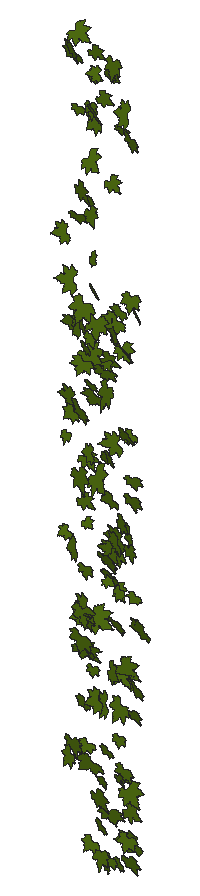
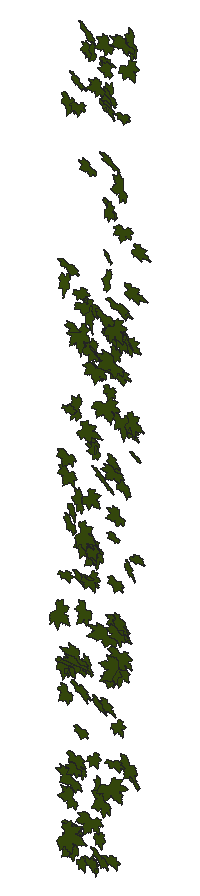
# SketchUp Ruby script. Lengths in inches.
U = 1.inch
M = Sketchup.active_model
def pt(a) = Geom::Point3d.new(a.map { |v| v * U })
def face(e, loops, mat)
  f = e.add_face(loops[0].map { |a| pt(a) })
  loops[1..].each { |l| e.add_face(l.map { |a| pt(a) }).erase! }
  f.material = f.back_material = mat if mat
  f
end
# faces: each face lists its corners as indices into pts; further lists are holes
def faces(e, pts, list, mat = nil) = list.each { |f| face(e, (f[0].is_a?(Array) ? f : [f]).map { |l| l.map { |i| pts[i] } }, mat) }
# xy, xz, yz: faces in a plane at the given z, y or x. An outline is a flat list of corners, or four numbers for a rectangle; further outlines are holes
def ring(l) = l.size == 4 ? [[l[0], l[1]], [l[2], l[1]], [l[2], l[3]], [l[0], l[3]]] : l.each_slice(2).to_a
def flat(e, list, mat, &to3) = list.each { |f| face(e, (f[0].is_a?(Array) ? f : [f]).map { |l| ring(l).map { |u, v| to3.(u, v) } }, mat) }
def xy(e, z, list, mat = nil) = flat(e, list, mat) { |x, y| [x, y, z] }
def xz(e, y, list, mat = nil) = flat(e, list, mat) { |x, z| [x, y, z] }
def yz(e, x, list, mat = nil) = flat(e, list, mat) { |y, z| [x, y, z] }
def lines(e, pts, list) = list.each { |a, b| e.add_line(pt(pts[a]), pt(pts[b])) }
# prism: a flat outline (further loops are holes) pulled along v
def prism(e, loops, v, mat = nil)
  f = face(e, loops, mat); d = Geom::Vector3d.new(v.map { |x| x * U })
  f.pushpull(f.normal.samedirection?(d) ? d.length : -d.length)
end
def box(e, o, s, mat = nil) = prism(e, [[o, [o[0] + s[0], o[1], o[2]], [o[0] + s[0], o[1] + s[1], o[2]], [o[0], o[1] + s[1], o[2]]]], [0, 0, s[2]], mat)
def at(x, y, z, deg = 0) = Geom::Transformation.translation(pt([x, y, z])) * Geom::Transformation.rotation(ORIGIN, Z_AXIS, deg.degrees)
def axes(o, x, y, z) = Geom::Transformation.new([*x, 0, *y, 0, *z, 0, *pt(o).to_a, 1])
def part(name) = M.definitions.add(name)
# library, detail: a bought-in or finely detailed component or shape, given as its bounding box
def library(name, o, s) = part(name).tap { |d| box(d.entities, o, s) }
def detail(e, o, s) = box(e.add_group.entities, o, s)
def put(e, d, t, mat = nil) = e.add_instance(d, t).tap { |i| i.material = mat if mat }
def group(e, t, mat = nil) = e.add_group.tap { |g| g.transformation = t; g.material = mat if mat }.entities
root = M.entities
M.materials.add("[Vegetation Blur 03]").color = [83, 114, 18]
c1 = part("ivy")
xy(c1.entities,0,[[0.782,0,0.786,0,0.787,0.005,0.789,0.009,0.821,0.072,0.875,0.147,1.001,0.272,1.073,0.331,1.137,0.363,1.178,0.379,1.223,0.384,1.272,0.383,1.311,0.374,1.36,0.355,1.399,0.334,1.491,0.285,1.541,0.244,1.583,0.199,1.617,0.15,1.64,0.128,1.662,0.115,1.717,0.105,1.745,0.093,1.784,0.054,1.819,0.057,1.854,0.064,1.882,0.075,1.896,0.074,1.91,0.071,1.937,0.063,1.964,0.053,1.99,0.038,2.016,0.015,2.034,0.002,2.04,0,2.038,0.003,2.036,0.007,2.033,0.038,2.036,0.068,2.045,0.1,2.055,0.116,2.064,0.123,2.077,0.129,2.088,0.129,2.106,0.132,2.118,0.13,2.179,0.132,2.207,0.133,2.225,0.133,2.242,0.138,2.22,0.162,2.207,0.186,2.206,0.213,2.212,0.236,2.228,0.262,2.247,0.274,2.298,0.283,2.355,0.294,2.37,0.296,2.376,0.295,2.377,0.3,2.377,0.303,2.385,0.329,2.411,0.37,2.426,0.392,2.449,0.407,2.511,0.426,2.561,0.444,2.619,0.466,2.589,0.469,2.561,0.476,2.501,0.5,2.449,0.516,2.424,0.523,2.401,0.535,2.377,0.556,2.372,0.568,2.36,0.575,2.268,0.586,2.225,0.592,2.207,0.599,2.194,0.61,2.143,0.65,2.13,0.664,2.122,0.682,2.123,0.7,2.13,0.719,2.148,0.75,2.17,0.781,2.195,0.807,2.221,0.828,2.284,0.874,2.291,0.88,2.288,0.887,2.276,0.9,2.267,0.916,2.265,0.933,2.273,0.967,2.292,1.002,2.313,1.03,2.334,1.054,2.348,1.067,2.358,1.074,2.363,1.076,2.362,1.081,2.35,1.094,2.347,1.11,2.35,1.143,2.359,1.18,2.385,1.254,2.415,1.324,2.448,1.393,2.45,1.4,2.446,1.398,2.44,1.394,2.427,1.383,2.402,1.36,2.376,1.339,2.345,1.324,2.305,1.309,2.282,1.303,2.273,1.306,2.245,1.294,2.212,1.287,2.187,1.291,2.163,1.301,2.142,1.316,2.134,1.327,2.124,1.325,2.09,1.292,2.053,1.259,2.014,1.234,1.973,1.215,1.954,1.21,1.931,1.208,1.909,1.212,1.893,1.22,1.879,1.233,1.872,1.248,1.867,1.281,1.864,1.319,1.821,1.258,1.773,1.197,1.726,1.141,1.698,1.121,1.679,1.116,1.666,1.117,1.647,1.122,1.632,1.129,1.62,1.141,1.617,1.154,1.617,1.219,1.621,1.254,1.623,1.268,1.623,1.281,1.618,1.314,1.606,1.346,1.603,1.375,1.607,1.403,1.603,1.467,1.599,1.499,1.605,1.525,1.614,1.552,1.629,1.577,1.635,1.589,1.629,1.587,1.618,1.582,1.596,1.566,1.581,1.556,1.568,1.552,1.557,1.55,1.545,1.553,1.531,1.562,1.522,1.572,1.504,1.591,1.486,1.611,1.474,1.631,1.457,1.666,1.455,1.684,1.457,1.698,1.452,1.715,1.444,1.728,1.424,1.754,1.419,1.772,1.423,1.786,1.434,1.819,1.444,1.848,1.446,1.855,1.44,1.861,1.43,1.867,1.386,1.904,1.349,1.948,1.326,1.973,1.31,1.995,1.288,2.048,1.284,2.153,1.287,2.254,1.284,2.255,1.282,2.253,1.278,2.247,1.274,2.237,1.266,2.216,1.226,2.125,1.208,2.076,1.184,2.033,1.155,1.984,1.135,1.942,1.111,1.899,1.083,1.861,1.053,1.85,1.059,1.83,1.061,1.809,1.056,1.79,1.049,1.767,1.04,1.749,1.018,1.733,0.994,1.726,0.942,1.734,0.95,1.6875,0.944,1.645,0.932,1.608,0.911,1.585,0.881,1.58,0.854,1.582,0.828,1.588,0.785,1.618,0.773,1.625,0.775,1.614,0.779,1.598,0.796,1.502,0.818,1.402,0.861,1.283,0.882,1.224,0.894,1.174,0.892,1.148,0.886,1.123,0.881,1.107,0.872,1.099,0.849,1.094,0.818,1.092,0.789,1.098,0.762,1.107,0.753,1.113,0.721,1.139,0.698,1.163,0.678,1.194,0.665,1.224,0.628,1.28,0.612,1.312,0.606,1.327,0.606,1.314,0.599,1.282,0.594,1.267,0.581,1.256,0.544,1.245,0.512,1.244,0.473,1.249,0.444,1.256,0.382,1.288,0.339,1.306,0.324,1.316,0.317,1.324,0.309,1.326,0.27,1.314,0.227,1.313,0.185,1.3125,0.152,1.317,0.122,1.328,0.092,1.345,0.073,1.353,0.079,1.338,0.092,1.308,0.117,1.249,0.13,1.215,0.139,1.164,0.147,1.148,0.157,1.136,0.163,1.122,0.174,1.086,0.177,1.067,0.182,1.054,0.186,1.043,0.191,1.038,0.211,1.028,0.237,1.005,0.25,0.974,0.253,0.96,0.25,0.944,0.242,0.914,0.243,0.906,0.249,0.902,0.26,0.894,0.289,0.88,0.307,0.873,0.322,0.862,0.364,0.799,0.403,0.738,0.431,0.709,0.439,0.691,0.441,0.678,0.4375,0.66,0.428,0.645,0.394,0.623,0.303,0.594,0.255,0.581,0.214,0.577,0.179,0.573,0.173,0.568,0.175,0.561,0.167,0.55,0.141,0.523,0.113,0.503,0.077,0.49,0.045,0.486,0.026,0.485,0.019,0.486,0.011,0.483,0,0.471,0.014,0.467,0.044,0.455,0.058,0.447,0.07,0.438,0.097,0.411,0.125,0.394,0.158,0.377,0.174,0.366,0.182,0.359,0.185,0.361,0.242,0.331,0.253,0.316,0.258,0.303,0.262,0.283,0.274,0.278,0.308,0.274,0.341,0.252,0.366,0.226,0.366,0.222,0.37,0.22,0.38,0.221,0.395,0.221,0.425,0.216,0.45,0.207,0.465,0.192,0.473,0.178,0.484,0.15,0.489,0.116,0.483,0.089,0.468,0.058,0.45,0.035,0.435,0.018,0.429,0.011,0.434,0.012,0.438,0.014,0.469,0.019,0.542,0.016,0.581,0.015,0.612,0.027,0.68,0.055,0.696,0.057,0.712,0.052,0.73,0.045,0.741,0.036,0.766,0.014]])
put(root,c1,axes([62.99,173.7,86.86],[0.22705,-0.11945,-0.35491],[-0.43835,-0.02,-0.18572],[-0.01818,-1.0093,0.04569]),"[Vegetation Blur 03]")
put(root,c1,axes([63.44,173.7,78.11],[0.07342,0.0201,-0.45241],[-0.55143,0.12193,-0.05876],[-0.05747,-1.14418,-0.01421]),"[Vegetation Blur 03]")
put(root,c1,axes([63,173.7,70.84],[0.22258,-0.06561,-0.19839],[-0.24493,-0.08915,-0.17839],[0.01076,-0.67235,0.04301]),"[Vegetation Blur 03]")
put(root,c1,axes([63.28,173.7,81.93],[0.13601,0.05917,-0.30855],[-0.37908,0.03752,-0.11017],[-0.00748,-0.82593,-0.02711]),"[Vegetation Blur 03]")
put(root,c1,axes([63.11,173.7,96.26],[0.33145,0.05992,-0.29685],[-0.36343,0.14447,-0.2657],[-0.03257,-1.00226,-0.05605]),"[Vegetation Blur 03]")
put(root,c1,axes([63.64,173.7,84.65],[0.1603,-0.20672,-0.46475],[-0.57787,-0.01388,-0.13179],[-0.02063,-1.21728,0.08043]),"[Vegetation Blur 03]")
put(root,c1,axes([62.82,173.7,75.76],[0.29106,-0.10296,0.03164],[0.02588,-0.14904,-0.23485],[-0.05776,-0.58557,0.05421]),"[Vegetation Blur 03]")
put(root,c1,axes([63.22,173.7,77.33],[0.3254,-0.08509,-0.21734],[-0.269,-0.05049,-0.26515],[-0.01633,-0.86378,0.03691]),"[Vegetation Blur 03]")
put(root,c1,axes([63.52,173.7,70.41],[0.27571,-0.25978,-0.33675],[-0.40528,0.18997,-0.24407],[-0.14812,-1.00337,0.04098]),"[Vegetation Blur 03]")
put(root,c1,axes([63.87,173.7,82.26],[0.12192,-0.00071,-0.41999],[-0.49465,0.29998,-0.09572],[-0.14193,-1.04612,-0.02717]),"[Vegetation Blur 03]")
put(root,c1,axes([63.06,173.7,59.27],[0.44114,-0.2833,-0.10477],[-0.14493,-0.08165,-0.37173],[-0.12012,-0.94191,0.06374]),"[Vegetation Blur 03]")
put(root,c1,axes([63.9,173.7,82.28],[0.14174,-0.20689,-0.42841],[-0.51411,0.25268,-0.13249],[-0.14609,-1.08996,0.0506]),"[Vegetation Blur 03]")
put(root,c1,axes([63.13,173.7,87.43],[0.38883,0.03177,-0.00541],[-0.00902,0.12865,-0.31342],[0.01417,-0.78985,-0.05127]),"[Vegetation Blur 03]")
put(root,c1,axes([63.375,173.7,93.22],[0.29737,0.00668,-0.03254],[-0.03987,-0.00069,-0.24271],[0.00326,-0.6174,-0.00008]),"[Vegetation Blur 03]")
put(root,c1,axes([63.875,173.7,66.67],[0.1748,-0.10036,-0.26156],[-0.32362,-0.01023,-0.14344],[-0.01895,-0.75115,0.0369]),"[Vegetation Blur 03]")
put(root,c1,axes([62.85,173.7,59.66],[0.54065,-0.21536,0.14176],[0.17436,-0.02611,-0.44914],[-0.10356,-1.16826,-0.01609]),"[Vegetation Blur 03]")
put(root,c1,axes([62.91,173.7,96.53],[0.22945,0.18892,0.3925],[0.48869,-0.02142,-0.18866],[0.02999,-1.09631,0.07132]),"[Vegetation Blur 03]")
put(root,c1,axes([63.86,173.7,82.72],[0.32489,0.11128,-0.34401],[-0.42351,0.17483,-0.25752],[-0.03505,-1.08109,-0.07706]),"[Vegetation Blur 03]")
put(root,c1,axes([63.32,173.7,77.73],[0.57169,-0.21875,-0.18427],[-0.21197,0.1873,-0.473],[-0.13171,-1.2509,-0.0386]),"[Vegetation Blur 03]")
put(root,c1,axes([62.86,173.7,96.42],[0.47356,-0.40672,0.26845],[0.33871,-0.06229,-0.41283],[-0.18036,-1.18486,-0.07045]),"[Vegetation Blur 03]")
put(root,c1,axes([63.83,173.7,62.08],[0.26898,-0.00531,-0.22272],[-0.27011,0.10743,-0.21769],[-0.03898,-0.78115,-0.02842]),"[Vegetation Blur 03]")
put(root,c1,axes([64.15,173.7,67.51],[0.26861,-0.16753,-0.42435],[-0.51691,0.14174,-0.22674],[-0.09889,-1.19591,0.03257]),"[Vegetation Blur 03]")
put(root,c1,axes([63.5,173.7,80.02],[0.48108,0.0091,-0.09014],[-0.10924,-0.11608,-0.39016],[0.0169,-1.00907,0.04407]),"[Vegetation Blur 03]")
put(root,c1,axes([63.25,173.7,65.55],[0.65346,-0.15996,-0.07236],[-0.08578,0.05992,-0.53686],[-0.0809,-1.3557,-0.01519]),"[Vegetation Blur 03]")
put(root,c1,axes([63.96,173.7,59.125],[0.44397,0.1395,-0.34863],[-0.43136,0.05055,-0.3627],[0.03168,-1.26682,-0.05286]),"[Vegetation Blur 03]")
put(root,c1,axes([63.92,173.7,64.72],[0.30297,0.01543,-0.16149],[-0.19571,0.1367,-0.2425],[-0.03016,-0.73198,-0.04869]),"[Vegetation Blur 03]")
put(root,c1,axes([63.91,173.7,59.875],[0.36198,-0.00364,-0.10329],[-0.12566,-0.10485,-0.29275],[0.01516,-0.7821,0.03972]),"[Vegetation Blur 03]")
put(root,c1,axes([64.55,173.7,88.52],[0.10541,0.02404,-0.33372],[-0.3979,0.2077,-0.08136],[-0.09494,-0.84377,-0.02954]),"[Vegetation Blur 03]")
put(root,c1,axes([63.51,173.7,72.11],[0.22933,0.01454,0.32661],[0.40022,0.004,-0.18721],[0.0052,-0.94915,0.00421]),"[Vegetation Blur 03]")
put(root,c1,axes([63.6875,173.7,69.01],[0.4011,-0.07198,0.04538],[0.05521,-0.01426,-0.32859],[-0.0356,-0.83315,0.0017]),"[Vegetation Blur 03]")
put(root,c1,axes([63.85,173.7,80.88],[0.3582,-0.18702,-0.03708],[-0.03384,0.10347,-0.29982],[-0.09581,-0.73577,-0.03274]),"[Vegetation Blur 03]")
put(root,c1,axes([63.33,173.7,66.79],[0.61675,-0.12461,0.11294],[0.13479,-0.08629,-0.50526],[-0.06818,-1.29784,0.02275]),"[Vegetation Blur 03]")
put(root,c1,axes([63.53,173.7,83.28],[0.64635,-0.1795,-0.0483],[-0.07498,-0.25102,-0.52154],[-0.0741,-1.31182,0.10641]),"[Vegetation Blur 03]")
put(root,c1,axes([63.16,173.7,64.34],[0.50593,-0.03643,0.3437],[0.41936,0.17969,-0.40818],[0.0424,-1.34262,-0.06395]),"[Vegetation Blur 03]")
put(root,c1,axes([64.57,173.7,75.52],[0.12968,-0.11784,-0.31424],[-0.38451,0.09135,-0.11108],[-0.06065,-0.83104,0.03235]),"[Vegetation Blur 03]")
put(root,c1,axes([63.5,173.7,66.26],[0.44883,-0.14962,0.17944],[0.22549,0.05754,-0.36812],[-0.05276,-1.02686,-0.04677]),"[Vegetation Blur 03]")
put(root,c1,axes([63.86,173.7,71.08],[0.14273,0.06127,0.20808],[0.25666,-0.04237,-0.11531],[-0.00355,-0.59977,0.0294]),"[Vegetation Blur 03]")
put(root,c1,axes([63.22,173.7,73.76],[0.52711,-0.21147,0.33505],[0.39283,-0.25745,-0.4372],[-0.15742,-1.35053,0.03088]),"[Vegetation Blur 03]")
put(root,c1,axes([63.56,173.7,74.49],[0.3729,0.07352,0.23123],[0.28448,-0.01242,-0.30497],[0.02479,-0.96364,0.02157]),"[Vegetation Blur 03]")
put(root,c1,axes([63.43,173.7,88.7],[0.32628,-0.20206,0.40603],[0.49033,-0.18475,-0.27691],[-0.12932,-1.21026,-0.02552]),"[Vegetation Blur 03]")
put(root,c1,axes([64.125,173.7,78.48],[0.49872,0.09657,-0.2358],[-0.29251,0.12066,-0.4043],[0.0109,-1.17989,-0.06065]),"[Vegetation Blur 03]")
put(root,c1,axes([64.25,173.7,54.9],[0.37574,-0.07096,-0.15978],[-0.19839,-0.07956,-0.3052],[-0.01253,-0.86822,0.04103]),"[Vegetation Blur 03]")
put(root,c1,axes([64.11,173.7,78.86],[0.33145,-0.08577,-0.02014],[-0.01771,0.11215,-0.26935],[-0.04508,-0.6747,-0.04221]),"[Vegetation Blur 03]")
put(root,c1,axes([63.47,173.7,79.82],[0.38163,0.10723,0.44815],[0.5511,-0.01709,-0.31195],[0.0229,-1.37595,0.0388]),"[Vegetation Blur 03]")
put(root,c1,axes([63.79,173.7,90.07],[0.21319,0.1755,0.40106],[0.49372,-0.23014,-0.15897],[-0.07069,-1.078,0.09923]),"[Vegetation Blur 03]")
put(root,c1,axes([64.23,173.7,63.84],[0.32221,-0.0387,0.02273],[0.02664,-0.04287,-0.26295],[-0.0205,-0.66413,0.01565]),"[Vegetation Blur 03]")
put(root,c1,axes([64.03,173.7,81.23],[0.32579,-0.0019,0.20222],[0.24053,-0.19974,-0.25841],[-0.05947,-0.81825,0.06261]),"[Vegetation Blur 03]")
put(root,c1,axes([64.35,173.7,85.17],[0.07732,0.04701,0.24249],[0.28519,-0.19481,-0.05463],[-0.0864,-0.60099,0.03668]),"[Vegetation Blur 03]")
put(root,c1,axes([65.03,173.7,95.72],[0.09099,-0.0894,-0.27257],[-0.33609,-0.07013,-0.07111],[0.02177,-0.70885,0.04141]),"[Vegetation Blur 03]")
put(root,c1,axes([64.1,173.7,93.6],[0.40522,-0.15446,0.13943],[0.15914,-0.15283,-0.3347],[-0.09744,-0.89194,0.0332]),"[Vegetation Blur 03]")
put(root,c1,axes([64.31,173.7,94.77],[0.07701,-0.01607,0.28736],[0.35217,-0.0014,-0.06288],[-0.00233,-0.74167,-0.00611]),"[Vegetation Blur 03]")
put(root,c1,axes([64.03,173.7,87.72],[0.34108,-0.07651,0.26436],[0.30846,-0.23678,-0.27587],[-0.10562,-0.93855,0.04805]),"[Vegetation Blur 03]")
put(root,c1,axes([64.86,173.7,62.86],[0.33179,-0.22508,-0.3253],[-0.40723,0.00189,-0.27687],[-0.0707,-1.0672,0.06812]),"[Vegetation Blur 03]")
put(root,c1,axes([63.87,173.7,65.75],[0.25598,0.2014,0.48378],[0.59803,0.04143,-0.21349],[0.05748,-1.32803,0.06671]),"[Vegetation Blur 03]")
put(root,c1,axes([64.6,173.7,93.49],[0.45619,-0.27219,-0.21417],[-0.27378,-0.03129,-0.38217],[-0.10679,-1.08253,0.0649]),"[Vegetation Blur 03]")
put(root,c1,axes([64.18,173.7,96.13],[0.23882,-0.04134,0.29544],[0.36225,0.06442,-0.19363],[0.01513,-0.89011,-0.02773]),"[Vegetation Blur 03]")
put(root,c1,axes([64.87,173.7,55.89],[0.29522,-0.08617,-0.18688],[-0.21829,0.16177,-0.24143],[-0.08083,-0.75161,-0.03054]),"[Vegetation Blur 03]")
put(root,c1,axes([64.54,173.7,83.73],[0.12614,-0.2409,0.28031],[0.3435,-0.16191,-0.12485],[-0.11696,-0.73532,-0.06434]),"[Vegetation Blur 03]")
put(root,c1,axes([64.125,173.7,82.33],[0.60257,-0.08021,0.1387],[0.16152,-0.21723,-0.48713],[-0.06569,-1.26991,0.07457]),"[Vegetation Blur 03]")
put(root,c1,axes([64.16,173.7,73.39],[0.26041,0.16269,0.49935],[0.59768,-0.40532,-0.18684],[-0.15294,-1.30696,0.1201]),"[Vegetation Blur 03]")
put(root,c1,axes([64.49,173.7,92.97],[0.11866,-0.26117,0.39663],[0.48542,-0.20436,-0.1179],[-0.12904,-1.00894,-0.07879]),"[Vegetation Blur 03]")
put(root,c1,axes([64.62,173.7,79.86],[0.50551,0.02715,-0.04471],[-0.05585,0.1053,-0.41049],[0.00753,-1.04102,-0.04269]),"[Vegetation Blur 03]")
put(root,c1,axes([65.2,173.7,59.91],[0.2455,0.02361,-0.20397],[-0.24867,0.10235,-0.19749],[-0.02754,-0.71362,-0.03507]),"[Vegetation Blur 03]")
put(root,c1,axes([65.43,173.7,62.82],[0.25932,-0.29593,-0.35358],[-0.43934,0.11655,-0.22996],[-0.12392,-1.03246,0.07539]),"[Vegetation Blur 03]")
put(root,c1,axes([65.24,173.7,70.6],[0.23892,0.03876,-0.2007],[-0.24369,0.14566,-0.1888],[-0.038,-0.69034,-0.0511]),"[Vegetation Blur 03]")
put(root,c1,axes([65.51,173.7,73.42],[0.22065,0.07279,-0.34055],[-0.41864,0.06201,-0.17859],[-0.01021,-0.96933,-0.037]),"[Vegetation Blur 03]")
put(root,c1,axes([64.6875,173.7,93.74],[0.16739,0.00231,0.3142],[0.38437,0.04772,-0.13645],[0.02172,-0.86254,-0.00671]),"[Vegetation Blur 03]")
put(root,c1,axes([65.25,173.7,69.24],[0.33471,0.047,-0.24757],[-0.30145,0.17573,-0.26622],[-0.0408,-0.91277,-0.064]),"[Vegetation Blur 03]")
put(root,c1,axes([64.79,173.7,58.03],[0.27088,-0.15261,0.15464],[0.19269,-0.01614,-0.22733],[-0.06536,-0.68006,-0.0293]),"[Vegetation Blur 03]")
put(root,c1,axes([64.33,173.7,57.01],[0.44693,-0.21309,0.34937],[0.42945,-0.06761,-0.37241],[-0.09772,-1.27172,-0.03874]),"[Vegetation Blur 03]")
put(root,c1,axes([64.65,173.7,54.41],[0.52824,-0.2088,0.07813],[0.0803,-0.17577,-0.43551],[-0.11407,-1.09065,0.05523]),"[Vegetation Blur 03]")
put(root,c1,axes([65.03,173.7,68.37],[0.12441,0.10653,0.22366],[0.27873,-0.02631,-0.1013],[0.00957,-0.61876,0.04281]),"[Vegetation Blur 03]")
put(root,c1,axes([65.2,173.7,54.22],[0.37274,-0.27698,-0.10257],[-0.11734,0.09274,-0.32343],[-0.14192,-0.80413,-0.00197]),"[Vegetation Blur 03]")
put(root,c1,axes([66.15,173.7,71.6],[0.10808,0.0782,-0.51354],[-0.62715,0.14615,-0.08441],[-0.06373,-1.30565,-0.04021]),"[Vegetation Blur 03]")
put(root,c1,axes([65.03,173.7,74.97],[0.1451,-0.1312,0.25798],[0.3214,0.00081,-0.12034],[-0.02623,-0.71573,-0.04743]),"[Vegetation Blur 03]")
put(root,c1,axes([65,173.7,80.03],[0.20968,0.01131,0.23173],[0.28004,-0.12895,-0.16779],[-0.0472,-0.71481,0.03394]),"[Vegetation Blur 03]")
put(root,c1,axes([65.25,173.7,70.875],[0.56655,-0.0115,-0.27779],[-0.34007,0.04247,-0.46224],[-0.01542,-1.35941,-0.01209]),"[Vegetation Blur 03]")
put(root,c1,axes([65.58,173.7,82.89],[0.41729,-0.27977,-0.39423],[-0.44817,0.37379,-0.3577],[-0.22574,-1.25924,-0.01859]),"[Vegetation Blur 03]")
put(root,c1,axes([64.79,173.7,56.41],[0.53014,0.02962,0.10212],[0.12282,0.12551,-0.4304],[0.02794,-1.11386,-0.04578]),"[Vegetation Blur 03]")
put(root,c1,axes([65.9375,173.7,71.35],[0.21226,-0.08156,-0.39258],[-0.47103,0.20087,-0.17619],[-0.10528,-1.06312,-0.00317]),"[Vegetation Blur 03]")
put(root,c1,axes([66.07,173.7,76.72],[0.17219,-0.03701,-0.43547],[-0.53302,-0.07752,-0.13935],[0.03036,-1.15115,0.02338]),"[Vegetation Blur 03]")
put(root,c1,axes([65.32,173.7,54.29],[0.37414,-0.10141,-0.07585],[-0.09511,-0.0243,-0.3074],[-0.04493,-0.79294,0.01912]),"[Vegetation Blur 03]")
put(root,c1,axes([64.73,173.7,69.96],[0.55336,-0.2755,0.17895],[0.23761,0.14136,-0.45516],[-0.0977,-1.21665,-0.0934]),"[Vegetation Blur 03]")
put(root,c1,axes([65,173.7,79.98],[0.16066,-0.07376,0.37357],[0.45903,0.04715,-0.13002],[0.00982,-0.99714,-0.03378]),"[Vegetation Blur 03]")
put(root,c1,axes([65.67,173.7,83.1],[0.38856,-0.00058,-0.29483],[-0.35992,-0.09405,-0.31593],[0.03091,-1.0877,0.02748]),"[Vegetation Blur 03]")
put(root,c1,axes([65.25,173.7,95.37],[0.16816,-0.15089,0.24654],[0.3088,-0.00002,-0.1403],[-0.03567,-0.71145,-0.05229]),"[Vegetation Blur 03]")
put(root,c1,axes([65.15,173.7,89.5],[0.24024,0.06291,0.29442],[0.3619,-0.06648,-0.19446],[-0.01006,-0.88941,0.03536]),"[Vegetation Blur 03]")
put(root,c1,axes([65.2,173.7,75.2],[0.23432,-0.21265,0.28086],[0.3439,-0.11223,-0.20448],[-0.10411,-0.84934,-0.0433]),"[Vegetation Blur 03]")
put(root,c1,axes([65.48,173.7,69.9],[0.13772,-0.02232,0.26418],[0.31478,-0.16115,-0.11144],[-0.07624,-0.70573,0.01709]),"[Vegetation Blur 03]")
put(root,c1,axes([65.7,173.7,81.74],[0.55985,-0.09656,-0.30764],[-0.35518,0.35678,-0.44814],[-0.13469,-1.34226,-0.09699]),"[Vegetation Blur 03]")
put(root,c1,axes([65.42,173.7,63.54],[0.07106,0.03212,0.39333],[0.4647,-0.27217,-0.05243],[-0.12873,-0.96482,0.02788]),"[Vegetation Blur 03]")
put(root,c1,axes([66.01,173.7,54.25],[0.22842,-0.06235,-0.19773],[-0.23665,0.11144,-0.18763],[-0.06007,-0.67607,-0.01269]),"[Vegetation Blur 03]")
put(root,c1,axes([65.92,173.7,83.52],[0.31144,-0.00755,-0.1936],[-0.23722,0.00118,-0.25419],[-0.00327,-0.80561,0.00144]),"[Vegetation Blur 03]")
put(root,c1,axes([65.19,173.7,79.39],[0.62306,-0.44776,0.08452],[0.0504,-0.33563,-0.52711],[-0.23565,-1.25564,0.11075]),"[Vegetation Blur 03]")
put(root,c1,axes([65.54,173.7,95.37],[0.14289,-0.07488,0.25812],[0.31299,-0.09737,-0.11985],[-0.0582,-0.70749,-0.01082]),"[Vegetation Blur 03]")
put(root,c1,axes([65.89,173.7,92.96],[0.30877,0.02964,-0.06253],[-0.07793,0.09874,-0.24894],[0.00225,-0.64717,-0.04084]),"[Vegetation Blur 03]")
put(root,c1,axes([65.39,173.7,96.48],[0.53111,-0.22481,0.11811],[0.12292,-0.23121,-0.43739],[-0.1333,-1.10892,0.06725]),"[Vegetation Blur 03]")
put(root,c1,axes([65.43,173.7,66.76],[0.46892,-0.24319,0.11777],[0.16224,0.13537,-0.38629],[-0.09203,-1.00049,-0.08089]),"[Vegetation Blur 03]")
put(root,c1,axes([65.76,173.7,60.71],[0.35341,-0.05372,0.02619],[0.03014,-0.05475,-0.28854],[-0.02834,-0.72817,0.01976]),"[Vegetation Blur 03]")
put(root,c1,axes([65.98,173.7,68.64],[0.31975,-0.13436,-0.03342],[-0.05173,-0.10756,-0.26163],[-0.05713,-0.65457,0.04985]),"[Vegetation Blur 03]")
put(root,c1,axes([65.79,173.7,58.5],[0.29444,-0.13699,0.14225],[0.1786,0.0132,-0.24425],[-0.05394,-0.70397,-0.03226]),"[Vegetation Blur 03]")
put(root,c1,axes([65.7,173.7,68.09],[0.20883,0.04815,0.31421],[0.37772,-0.20796,-0.1622],[-0.0781,-0.87697,0.05572]),"[Vegetation Blur 03]")
put(root,c1,axes([67.03,173.7,55.86],[0.10967,0.16764,-0.53959],[-0.66571,-0.0227,-0.09123],[0.02429,-1.37893,-0.0641]),"[Vegetation Blur 03]")
put(root,c1,axes([66.83,173.7,94.43],[0.1383,-0.27518,-0.42018],[-0.52123,0.14835,-0.12955],[-0.10615,-1.08693,0.0887]),"[Vegetation Blur 03]")
put(root,c1,axes([65.5,173.7,63.87],[0.43423,0.11965,0.28912],[0.35873,-0.10053,-0.35232],[0.01383,-1.14881,0.06094]),"[Vegetation Blur 03]")
put(root,c1,axes([65.9,173.7,62.91],[0.58633,-0.27865,-0.1062],[-0.1477,-0.14213,-0.48453],[-0.11598,-1.22771,0.08019]),"[Vegetation Blur 03]")
put(root,c1,axes([65.73,173.7,80.98],[0.34318,0.09184,0.26358],[0.326,-0.10859,-0.27677],[-0.00403,-0.96364,0.05631]),"[Vegetation Blur 03]")
put(root,c1,axes([65.97,173.7,59.3],[0.4987,-0.12613,-0.04723],[-0.0598,-0.02572,-0.40975],[-0.05942,-1.03278,0.01597]),"[Vegetation Blur 03]")
put(root,c1,axes([65.99,173.7,58.47],[0.24944,0.02336,0.19362],[0.23616,0.05082,-0.20362],[0.02524,-0.70655,-0.00824]),"[Vegetation Blur 03]")
put(root,c1,axes([66.67,173.7,63.9],[0.17883,0.01791,-0.19414],[-0.23754,0.05276,-0.14498],[-0.01529,-0.61012,-0.01823]),"[Vegetation Blur 03]")
put(root,c1,axes([65.57,173.7,63.91],[0.34678,0.03788,0.46084],[0.56412,0.05104,-0.28341],[0.03077,-1.36263,0.00219]),"[Vegetation Blur 03]")
put(root,c1,axes([65.98,173.7,71.81],[0.1731,-0.14266,0.38005],[0.45428,-0.21748,-0.15066],[-0.12362,-0.99891,-0.02148]),"[Vegetation Blur 03]")
put(root,c1,axes([66.625,173.7,72.12],[0.31941,-0.24553,-0.21108],[-0.24847,0.1507,-0.27802],[-0.13923,-0.8322,0.01193]),"[Vegetation Blur 03]")
put(root,c1,axes([66.19,173.7,55.7],[0.48615,-0.06506,-0.03255],[-0.04363,-0.12709,-0.39413],[-0.0262,-0.99568,0.05243]),"[Vegetation Blur 03]")
put(root,c1,axes([66.68,173.7,77.18],[0.29981,-0.06525,-0.13535],[-0.1686,-0.07812,-0.24283],[-0.00912,-0.70071,0.03968]),"[Vegetation Blur 03]")
put(root,c1,axes([66.19,173.7,76.49],[0.13916,-0.21976,0.37305],[0.46529,-0.06512,-0.12164],[-0.06205,-0.98109,-0.07549]),"[Vegetation Blur 03]")
put(root,c1,axes([67.36,173.7,67.15],[0.17288,0.13727,-0.46997],[-0.57483,0.20036,-0.13164],[-0.0749,-1.22089,-0.07445]),"[Vegetation Blur 03]")
put(root,c1,axes([66.38,173.7,74.55],[0.40772,-0.01716,0.08723],[0.10718,0.04684,-0.33224],[-0.00228,-0.8661,-0.01969]),"[Vegetation Blur 03]")
put(root,c1,axes([66.82,173.7,68.62],[0.28445,-0.01133,-0.1134],[-0.139,-0.04223,-0.23156],[0.00407,-0.65007,0.01702]),"[Vegetation Blur 03]")
put(root,c1,axes([66.75,173.7,83.88],[0.40706,-0.21039,-0.21028],[-0.21941,0.3311,-0.33502],[-0.1694,-0.93442,-0.07136]),"[Vegetation Blur 03]")
put(root,c1,axes([66.34,173.7,84.3125],[0.49447,-0.06651,0.04707],[0.05156,-0.17262,-0.39913],[-0.04138,-1.00977,0.06513]),"[Vegetation Blur 03]")
put(root,c1,axes([66.41,173.7,92.84],[0.50217,-0.23211,-0.02067],[-0.01614,0.08923,-0.41886],[-0.11447,-1.03084,-0.03161]),"[Vegetation Blur 03]")
put(root,c1,axes([65.95,173.7,57.65],[0.43574,0.04341,0.40329],[0.4922,-0.17124,-0.35133],[-0.04861,-1.34487,0.05775]),"[Vegetation Blur 03]")
put(root,c1,axes([66.26,173.7,56.53],[0.18345,-0.01602,0.41607],[0.50825,-0.08298,-0.14976],[-0.04057,-1.11184,0.00518]),"[Vegetation Blur 03]")
put(root,c1,axes([66.16,173.7,54.36],[0.49317,-0.18476,0.20262],[0.2548,0.0498,-0.40595],[-0.06909,-1.1351,-0.05079]),"[Vegetation Blur 03]")
put(root,c1,axes([66.34,173.7,73.625],[0.48848,-0.12647,0.08295],[0.10536,0.05262,-0.40062],[-0.05484,-1.02537,-0.03079]),"[Vegetation Blur 03]")
put(root,c1,axes([66.38,173.7,70.84],[0.37427,-0.16845,0.18276],[0.21743,-0.11081,-0.31265],[-0.09784,-0.89065,0.00433]),"[Vegetation Blur 03]")
put(root,c1,axes([66.75,173.7,63.94],[0.464,-0.18688,-0.09777],[-0.10719,0.14954,-0.38378],[-0.10541,-0.97473,-0.04013]),"[Vegetation Blur 03]")
put(root,c1,axes([66.52,173.7,62.15],[0.36419,-0.14328,0.1768],[0.2225,0.04791,-0.29916],[-0.04769,-0.87068,-0.04556]),"[Vegetation Blur 03]")
